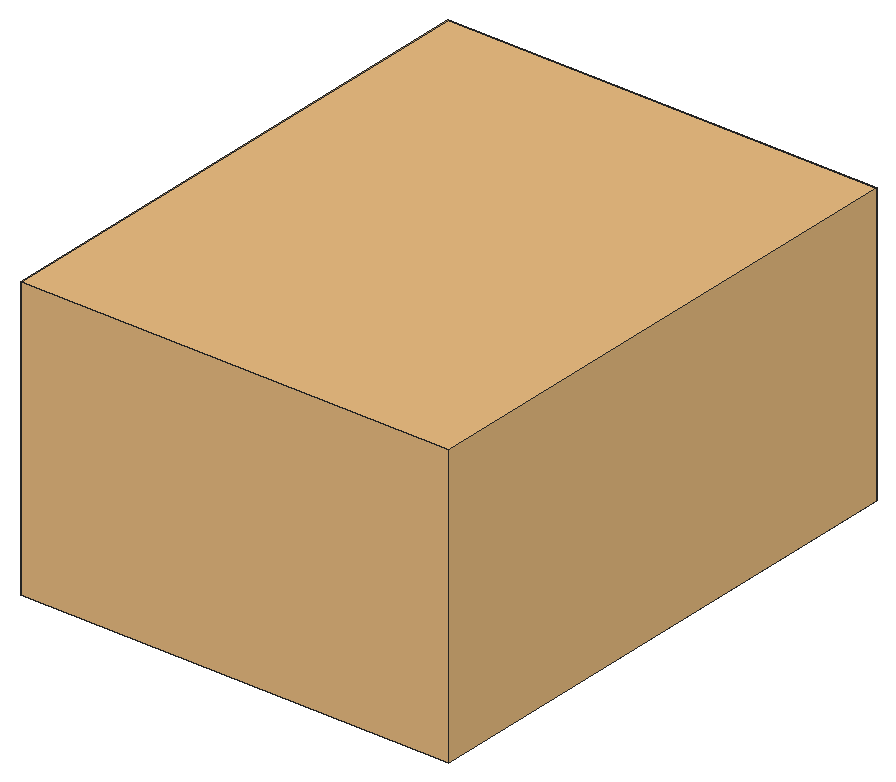
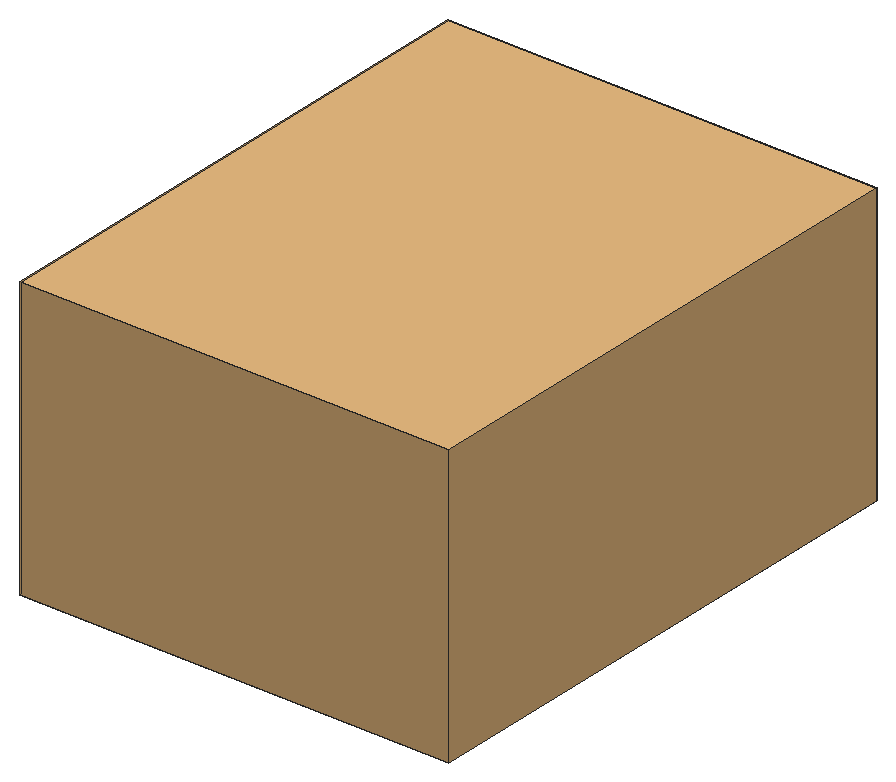
# SketchUp Ruby script. Lengths in inches.
U = 1.inch
M = Sketchup.active_model
def pt(a) = Geom::Point3d.new(a.map { |v| v * U })
def face(e, loops, mat)
  f = e.add_face(loops[0].map { |a| pt(a) })
  loops[1..].each { |l| e.add_face(l.map { |a| pt(a) }).erase! }
  f.material = f.back_material = mat if mat
  f
end
# faces: each face lists its corners as indices into pts; further lists are holes
def faces(e, pts, list, mat = nil) = list.each { |f| face(e, (f[0].is_a?(Array) ? f : [f]).map { |l| l.map { |i| pts[i] } }, mat) }
# xy, xz, yz: faces in a plane at the given z, y or x. An outline is a flat list of corners, or four numbers for a rectangle; further outlines are holes
def ring(l) = l.size == 4 ? [[l[0], l[1]], [l[2], l[1]], [l[2], l[3]], [l[0], l[3]]] : l.each_slice(2).to_a
def flat(e, list, mat, &to3) = list.each { |f| face(e, (f[0].is_a?(Array) ? f : [f]).map { |l| ring(l).map { |u, v| to3.(u, v) } }, mat) }
def xy(e, z, list, mat = nil) = flat(e, list, mat) { |x, y| [x, y, z] }
def xz(e, y, list, mat = nil) = flat(e, list, mat) { |x, z| [x, y, z] }
def yz(e, x, list, mat = nil) = flat(e, list, mat) { |y, z| [x, y, z] }
def lines(e, pts, list) = list.each { |a, b| e.add_line(pt(pts[a]), pt(pts[b])) }
# prism: a flat outline (further loops are holes) pulled along v
def prism(e, loops, v, mat = nil)
  f = face(e, loops, mat); d = Geom::Vector3d.new(v.map { |x| x * U })
  f.pushpull(f.normal.samedirection?(d) ? d.length : -d.length)
end
def box(e, o, s, mat = nil) = prism(e, [[o, [o[0] + s[0], o[1], o[2]], [o[0] + s[0], o[1] + s[1], o[2]], [o[0], o[1] + s[1], o[2]]]], [0, 0, s[2]], mat)
def at(x, y, z, deg = 0) = Geom::Transformation.translation(pt([x, y, z])) * Geom::Transformation.rotation(ORIGIN, Z_AXIS, deg.degrees)
def axes(o, x, y, z) = Geom::Transformation.new([*x, 0, *y, 0, *z, 0, *pt(o).to_a, 1])
def part(name) = M.definitions.add(name)
# library, detail: a bought-in or finely detailed component or shape, given as its bounding box
def library(name, o, s) = part(name).tap { |d| box(d.entities, o, s) }
def detail(e, o, s) = box(e.add_group.entities, o, s)
def put(e, d, t, mat = nil) = e.add_instance(d, t).tap { |i| i.material = mat if mat }
def group(e, t, mat = nil) = e.add_group.tap { |g| g.transformation = t; g.material = mat if mat }.entities
root = M.entities
M.materials.add("D02_Buttercup_Glow").color = [255, 229, 155]
M.materials.add("LightPink_Translucent").color = [144, 107, 117]
c1 = part("blade")
p = [[2.15,0.21,22],[0,0.17,0],[0.09,0.45,0],[2.18,0.31,22],[2.29,0.31,22],[0.38,0.45,0],
  [2.48,0.24,33],[2.49,0.24,33],[2.48,0.22,33]]
faces(c1.entities,p,[[0,1,2,3],[4,5,2,3],[6,3,4,7],[8,0,3,6]])
c2 = part("seeds")
p = [[0.3,-0.1,1.38],[-0.01,-0.03,1.59],[-0.01,-0.03,0.03],[0.14,-0.07,-0.07],[0.29,-0.03,3],[0.15,0.01,3.11]]
faces(c2.entities,p,[[0,1,2,3],[1,0,4,5]],"LightPink_Translucent")
c3 = part("blade with seeds")
put(c3.entities,c1,at(0,0,0))
put(c3.entities,c2,axes([2.4,0.25,30.99],[1.5799,-0.05474,1.17369],[-0.12525,1.92788,0.29478],[-0.07173,-0.02425,1.56792]))
c4 = library("Group\#1",[297.81,-2,0],[578,722,378])
put(root,c3,axes([77.12,76.59,44.18],[1.2866,-0.3514,-0.19198],[0.45209,1.01223,0.00008],[0.14202,-0.03884,1.73897]))
put(root,c3,axes([65.8,73.25,44.06],[1.27479,0.1698,-0.62353],[-0.26901,1.04736,-0.16365],[0.38043,0.12691,1.37633]))
put(root,c3,axes([77.8,73.25,44.06],[1.27479,0.1698,-0.62353],[-0.26901,1.04736,-0.16365],[0.38043,0.12691,1.37633]))
put(root,c3,axes([64.37,75.88,44.46],[-1.19666,-0.83357,-0.25192],[1.00694,-0.93603,0.5513],[-0.32224,0.09751,1.68216]))
put(root,c3,axes([76.37,75.88,44.46],[-1.19666,-0.83357,-0.25192],[1.00694,-0.93603,0.5513],[-0.32224,0.09751,1.68216]))
put(root,c3,axes([65.14,73.58,44.21],[0.73619,0.86927,-0.44739],[-1.11511,0.61213,0.21531],[0.23824,0.10756,1.43643]))
put(root,c3,axes([77.14,73.58,44.21],[0.73619,0.86927,-0.44739],[-1.11511,0.61213,0.21531],[0.23824,0.10756,1.43643]))
put(root,c3,axes([63.76,75.7,44.21],[-1.33077,0.06393,-0.44739],[-0.12035,-1.06125,0.21531],[-0.23824,0.10756,1.43643]))
put(root,c3,axes([75.76,75.7,44.21],[-1.33077,0.06393,-0.44739],[-0.12035,-1.06125,0.21531],[-0.23824,0.10756,1.43643]))
put(root,c3,axes([64.89,78.03,44.03],[-1.14332,-0.25625,-0.30978],[0.28787,-0.90242,0.30978],[-0.23049,0.10406,1.38974]))
put(root,c3,axes([76.89,78.03,44.03],[-1.14332,-0.25625,-0.30978],[0.28787,-0.90242,0.30978],[-0.23049,0.10406,1.38974]))
put(root,c3,axes([65.38,74.18,44.67],[1.38012,0.49416,-0.29095],[-0.66454,1.04299,-0.50002],[0.04337,0.25608,1.59708]))
put(root,c3,axes([77.38,74.18,44.67],[1.38012,0.49416,-0.29095],[-0.66454,1.04299,-0.50002],[0.04337,0.25608,1.59708]))
put(root,c3,axes([68.38,75.35,44.03],[-0.85545,0.64616,-0.30978],[-0.85545,-0.64616,0.30978],[0,0.20813,1.38974]))
put(root,c3,axes([80.38,75.35,44.03],[-0.85545,0.64616,-0.30978],[-0.85545,-0.64616,0.30978],[0,0.20813,1.38974]))
put(root,c3,axes([64.69,75.42,44.67],[0.1428,1.18174,-0.29095],[-1.48733,0.07145,-0.50002],[-0.26191,0.15741,1.59708]))
put(root,c3,axes([76.69,75.42,44.67],[0.1428,1.18174,-0.29095],[-1.48733,0.07145,-0.50002],[-0.26191,0.15741,1.59708]))
put(root,c3,axes([65.24,74.95,44.21],[-0.59459,0.93321,-0.44739],[-1.23546,-0.44912,0.21531],[0,0.21512,1.43643]))
put(root,c3,axes([77.24,74.95,44.21],[-0.59459,0.93321,-0.44739],[-1.23546,-0.44912,0.21531],[0,0.21512,1.43643]))
put(root,c3,axes([63.8,76.32,44.06],[-0.82544,0.77843,-0.62353],[-1.0254,-0.70586,-0.16365],[-0.33076,0.19418,1.37633]))
put(root,c3,axes([75.8,76.32,44.06],[-0.82544,0.77843,-0.62353],[-1.0254,-0.70586,-0.16365],[-0.33076,0.19418,1.37633]))
put(root,c3,axes([65.16,78.44,44.02],[-1.14694,0.51783,-0.49651],[-0.68554,-0.92854,0],[-0.26122,0.11794,1.57504]))
put(root,c3,axes([77.16,78.44,44.02],[-1.14694,0.51783,-0.49651],[-0.68554,-0.92854,0],[-0.26122,0.11794,1.57504]))
put(root,c3,axes([68.97,75.38,44.02],[0,1.03566,-0.49651],[-1.37109,0,0],[0,0.23588,1.57504]))
put(root,c3,axes([80.97,75.38,44.02],[0,1.03566,-0.49651],[-1.37109,0,0],[0,0.23588,1.57504]))
put(root,c3,axes([67.42,78.63,43.49],[0.08928,-0.14952,1.76342],[1.12407,-0.44035,-0.26939],[0.34078,0.22791,0.30037]))
put(root,c3,axes([79.42,78.63,43.49],[0.08928,-0.14952,1.76342],[1.12407,-0.44035,-0.26939],[0.34078,0.22791,0.30037]))
put(root,c3,axes([65.94,75.24,44.09],[0.44936,0.94823,-0.69212],[-1.29441,0.3415,-0.18165],[0.04967,0.32109,1.52773]))
put(root,c3,axes([77.94,75.24,44.09],[0.44936,0.94823,-0.69212],[-1.29441,0.3415,-0.18165],[0.04967,0.32109,1.52773]))
put(root,c3,axes([57.1,78.51,43.49],[0.16438,0.10347,1.76342],[0.27873,0.95868,-0.26939],[-0.36432,0.20444,0.30037]))
put(root,c3,axes([69.1,78.51,43.49],[0.16438,0.10347,1.76342],[0.27873,0.95868,-0.26939],[-0.36432,0.20444,0.30037]))
put(root,c3,axes([62.17,78.6,43.49],[0.19833,-0.05635,1.76342],[1.19302,0.31018,-0.26939],[0.03489,0.3496,0.30037]))
put(root,c3,axes([74.17,78.6,43.49],[0.19833,-0.05635,1.76342],[1.19302,0.31018,-0.26939],[0.03489,0.3496,0.30037]))
put(root,c4,at(-770.92,3.11,-6),"D02_Buttercup_Glow")
put(root,c3,axes([72.59,385.52,32.11],[0.28013,0.33252,1.71376],[-1.29445,0.27994,0.13857],[-0.29256,-0.52202,0.73262]))
put(root,c3,axes([74.73,383.31,32.95],[-0.18744,-0.14521,1.74944],[-1.25089,0.09206,-0.27667],[-0.19964,-0.34731,0.14031]))
put(root,c3,axes([77.625,385.04,30.83],[-0.34835,0.20963,1.43002],[-1.04325,-0.36691,-0.30754],[0.19338,-0.4563,0.61141]))
put(root,c3,axes([76.04,385.77,33.22],[-0.5849,-0.8421,-0.71045],[1.20401,-0.4693,0.08574],[-0.13677,-0.40688,1.00501]))
put(root,c3,axes([72.23,384.64,30.83],[-0.07421,0.33879,1.43002],[-1.08488,0.28361,-0.30754],[-0.25359,-0.4379,0.61141]))
put(root,c3,axes([75.03,383.9,29.73],[-0.20555,0.03731,1.76342],[-1.13672,-0.42002,-0.26939],[0.01907,-0.35034,0.30037]))
put(root,c3,axes([78.47,386.59,33.22],[0.03189,-0.95798,-0.71045],[1.34277,0.06434,0.08574],[0.14171,-0.40585,1.00501]))
put(root,c3,axes([80.35,385.09,32.95],[-0.01183,-0.20612,1.74944],[-0.99913,-0.59572,-0.27667],[0.15447,-0.36112,0.14031]))
put(root,c3,axes([76.15,385.05,32.76],[0.36946,-0.79643,-0.35414],[1.07787,0.23229,0.4572],[-0.09883,-0.32066,0.87481]))
put(root,c3,axes([76.96,386.11,32.11],[-0.22818,0.35597,1.71376],[-0.95725,-0.73667,0.13857],[0.43183,-0.45914,0.73262]))
put(root,c3,axes([80.08,384.35,32.95],[-0.12446,0.07911,1.77383],[-1.21937,-0.26689,-0.16761],[-0.04414,-0.34521,0.31391]))
put(root,c3,axes([75.6,385.6,32.92],[-1.20468,-0.25962,-0.51099],[0.41292,-0.89013,-0.3958],[-0.11046,-0.35838,0.97773]))
put(root,c3,axes([76.34,383.37,31],[0.15721,0.60392,1.1486],[-0.87211,-0.33448,0.84392],[0.09385,-0.30923,0.25299]))
put(root,c3,axes([78.2,386.27,32.92],[-0.87728,-0.69587,-0.51099],[0.92674,-0.60943,-0.3958],[0.13348,-0.35356,0.97773]))
put(root,c3,axes([73.44,382.84,32.95],[-0.02286,0.12414,1.77383],[-1.12758,0.45052,-0.16761],[-0.33182,-0.23029,0.31391]))
put(root,c3,axes([73.2,385.04,33.33],[1.36515,-0.26619,0.53763],[0.23692,1.04421,0.4433],[-0.32106,-0.30775,1.11249]))
put(root,c3,axes([76.28,385.24,32.97],[1.20755,0.27075,0.48003],[-0.41292,0.89013,0.3958],[-0.07257,-0.35005,0.9933]))
put(root,c3,axes([76.63,385.56,33.27],[-1.19922,0.48218,-0.1216],[-0.58932,-0.85579,-0.67495],[-0.15822,-0.36063,1.02557]))
put(root,c3,axes([79.12,386.64,33.27],[-1.34686,-0.05131,-0.1216],[0.03681,-0.97156,-0.67495],[0.09356,-0.37418,1.02557]))
put(root,c3,axes([79.03,386.01,32.76],[0.82919,-0.54528,-0.35414],[0.78493,0.62262,0.4572],[0.11943,-0.31634,0.87481]))
put(root,c3,axes([71.86,384.09,31],[0.63926,0.36046,1.1486],[-0.93099,0.21668,0.84392],[-0.1992,-0.27702,0.25299]))
put(root,c3,axes([76.6,385.17,32.97],[0.90301,-0.35198,0.0643],[0.44199,0.64184,0.50621],[-0.08721,-0.28293,0.77189]))
put(root,c3,axes([73.4,386.01,33.22],[-1.04497,-0.50058,-0.71045],[0.74264,-0.8772,0.08574],[-0.3786,-0.29889,1.00501]))
put(root,c3,axes([73.04,385.34,32.76],[-0.18927,-0.83419,-0.35414],[1.08199,-0.22027,0.4572],[-0.29062,-0.23905,0.87481]))
put(root,c3,axes([73.51,385.27,32.97],[0.55698,-0.6579,0.0643],[0.79316,0.38303,0.50621],[-0.25643,-0.21093,0.77189]))
put(root,c3,axes([71.35,385.18,29.73],[-0.11871,0.13643,1.76342],[-1.19964,0.29415,-0.26939],[-0.2898,-0.26759,0.30037]))
put(root,c3,axes([34.1875,387.14,43.49],[-0.20555,0.03731,1.76342],[-1.13672,-0.42002,-0.26939],[0.01907,-0.35034,0.30037]))
put(root,c3,axes([73.33,388.93,30.33],[-0.50328,-1.06202,-0.69835],[1.44974,-0.38248,-0.18329],[-0.05563,-0.35963,1.54149]))
put(root,c3,axes([70.71,386.56,32.11],[0.45521,0.17844,1.71376],[-0.94204,0.74856,0.13857],[-0.58713,-0.33769,0.73262]))
put(root,c3,axes([80.0625,385.69,29.73],[-0.18342,-0.08159,1.76342],[-0.47115,-0.9115,-0.26939],[0.31784,-0.24736,0.30037]))
put(root,c3,axes([76.27,385.89,33.29],[-0.36946,0.79643,0.35414],[-1.07787,-0.23229,-0.4572],[-0.09883,-0.32066,0.87481]))
put(root,c3,axes([72.91,386.03,32.92],[-1.20928,0.24619,-0.51099],[-0.21154,-0.93233,-0.3958],[-0.32481,-0.26718,0.97773]))
put(root,c3,axes([79.02,386.23,32.97],[0.87265,0.70663,0.48003],[-0.92674,0.60943,0.3958],[0.16097,-0.33153,0.9933]))
put(root,c3,axes([73.76,385.2,33.67],[-0.81789,0.99285,-0.13619],[-1.18445,-0.572,-0.75594],[-0.41173,-0.28051,1.14864]))
put(root,c3,axes([79.35,386.29,32.97],[1.00708,0.04826,0.0643],[-0.02761,0.72867,0.50621],[0.10538,-0.27912,0.77189]))
put(root,c3,axes([78.59,386.79,33.29],[-0.82919,0.54528,0.35414],[-0.78493,-0.62262,-0.4572],[0.11943,-0.31634,0.87481]))
put(root,c3,axes([80.06,388.26,33.22],[0.64013,-0.81717,-0.71045],[1.12174,0.58074,0.08574],[0.38221,-0.29607,1.00501]))
put(root,c3,axes([73.14,385.875,30.61],[-0.7662,-1.03778,0],[1.28187,-0.57875,-0.51607],[0.29196,-0.13181,1.63711]))
put(root,c3,axes([80.02,387.875,32.92],[-0.31482,-0.94565,-0.51099],[1.19224,-0.16542,-0.3958],[0.34166,-0.254,0.97773]))
put(root,c3,axes([74.82,384.625,30.36],[-0.84686,0.59414,-0.03893],[-0.77596,-0.65071,-0.17649],[-0.05463,-0.18438,0.58215]))
put(root,c3,axes([70.625,384.91,32.95],[-0.26368,-0.00731,1.74944],[-0.83946,0.73103,-0.27667],[-0.44791,-0.14937,0.14031]))
put(root,c3,axes([80.59,388.55,33.27],[-1.1336,-0.57106,-0.1216],[0.65308,-0.827,-0.67495],[0.32027,-0.28747,1.02557]))
put(root,c3,axes([75.9,391.67,31.5625],[1.05902,0.41762,1.51261],[-1.03748,0.89969,0.59816],[-0.46471,-0.53324,1.26806]))
put(root,c3,axes([73.68,386.02,33.29],[0.18927,0.83419,0.35414],[-1.08199,0.22027,-0.4572],[-0.29062,-0.23905,0.87481]))
put(root,c3,axes([70.37,388.78,30.25],[0,-1.03566,-0.49651],[1.37109,0,0],[0,-0.23588,1.57504]))
put(root,c3,axes([74.18,385.72,30.25],[1.14694,-0.51783,-0.49651],[0.68554,0.92854,0],[0.26122,-0.11794,1.57504]))
put(root,c3,axes([80.98,387.51,30.83],[-0.4378,-0.03068,1.43002],[-0.44851,-0.8229,-0.30754],[0.53783,-0.23279,0.61141]))
put(root,c3,axes([70.43,386.57,33.33],[1.01205,-0.7643,0.53763],[0.87284,0.81167,0.4433],[-0.47482,-0.14098,1.11249]))
put(root,c3,axes([83.38,388.3,32.95],[-0.16006,-0.00787,1.77383],[-0.66468,-0.8428,-0.16761],[0.26693,-0.27711,0.31391]))
put(root,c3,axes([75.54,387.84,30.3],[0.82544,-0.77843,-0.62353],[1.0254,0.70586,-0.16365],[0.33076,-0.19418,1.37633]))
put(root,c3,axes([81.49,385.99,31],[-0.40819,0.5272,1.1486],[-0.35086,-0.70831,0.84392],[0.33713,-0.17749,0.25299]))
put(root,c3,axes([80.9,387.97,32.76],[1.06674,-0.14801,-0.35414],[0.28168,0.84611,0.4572],[0.30569,-0.22726,0.87481]))
put(root,c3,axes([30.51,388.42,43.49],[-0.11871,0.13643,1.76342],[-1.19964,0.29415,-0.26939],[-0.2898,-0.26759,0.30037]))
put(root,c3,axes([70.89,386.5625,32.97],[0.06171,-0.78753,0.0643],[0.9318,0.02159,0.50621],[-0.35694,-0.08241,0.77189]))
put(root,c3,axes([32.49,392.17,44.1],[-0.50328,-1.06202,-0.69835],[1.44974,-0.38248,-0.18329],[-0.05563,-0.35963,1.54149]))
put(root,c3,axes([74.1,389.2,30.45],[0.59459,-0.93321,-0.44739],[1.23546,0.44912,0.21531],[0,-0.21512,1.43643]))
put(root,c3,axes([70.54,386.8125,32.76],[-0.69728,-0.64842,-0.35414],[0.79619,-0.61382,0.4572],[-0.40453,-0.09339,0.87481]))
put(root,c3,axes([39.22,388.93,43.49],[-0.18342,-0.08159,1.76342],[-0.47115,-0.9115,-0.26939],[0.31784,-0.24736,0.30037]))
put(root,c3,axes([74.64,388.74,30.9],[-0.1428,-1.18174,-0.29095],[1.48733,-0.07145,-0.50002],[0.26191,-0.15741,1.59708]))
put(root,c3,axes([70.95,388.8,30.26],[0.85545,-0.64616,-0.30978],[0.85545,0.64616,0.30978],[0,-0.20813,1.38974]))
put(root,c3,axes([70.61,385.71,30.36],[-0.35352,0.84566,-0.03893],[-1.08806,-0.26014,-0.17649],[-0.1652,-0.13832,0.58215]))
put(root,c3,axes([80.03,388.47,33.29],[-1.06674,0.14801,0.35414],[-0.28168,-0.84611,-0.4572],[0.30569,-0.22726,0.87481]))
put(root,c3,axes([73.95,389.98,30.9],[-1.38012,-0.49416,-0.29095],[0.66454,-1.04299,-0.50002],[-0.04337,-0.25608,1.59708]))
put(root,c3,axes([70.02,389.57,30.61],[-1.53239,0,0],[0,-1.1575,-0.51607],[0,-0.26363,1.63711]))
put(root,c3,axes([70.29,387.5,30.83],[0.23927,0.28834,1.43002],[-0.55135,0.78376,-0.30754],[-0.56612,-0.18733,0.61141]))
put(root,c3,axes([74.45,386.125,30.26],[1.14332,0.25625,-0.30978],[-0.28787,0.90242,0.30978],[0.23049,-0.10406,1.38974]))
put(root,c3,axes([71.27,387.24,33.22],[-1.22504,-0.02494,-0.71045],[0.08228,-1.05005,0.08574],[-0.51899,-0.11081,1.00501]))
put(root,c3,axes([33.98,387.87,44.13],[-0.84686,0.59414,-0.03893],[-0.77596,-0.65071,-0.17649],[-0.05463,-0.18438,0.58215]))
put(root,c3,axes([81,388.34,32.97],[0.8413,0.43556,0.0643],[-0.48981,0.62025,0.50621],[0.26973,-0.20053,0.77189]))
put(root,c3,axes([80.77,388.16,32.97],[0.30393,0.95317,0.48003],[-1.19224,0.16542,0.3958],[0.35138,-0.22417,0.9933]))
put(root,c3,axes([83.98,389.31,32.95],[0.17006,-0.15775,1.74944],[-0.21766,-0.96766,-0.27667],[0.42669,-0.18347,0.14031]))
put(root,c3,axes([71.21,389.26,30.57],[-1.1399,0.87071,0.30756],[-1.1406,-0.86155,-0.36492],[-0.03981,-0.24727,1.64885]))
put(root,c3,axes([69.61,385.53,32.95],[0.09085,0.10335,1.77383],[-0.43798,0.92907,-0.16761],[-0.44357,0.00672,0.31391]))
put(root,c3,axes([74.84,389.67,30.67],[1.3808,0.50196,0.24065],[-0.66454,1.04299,0.50002],[0,-0.24043,1.60543]))
put(root,c3,axes([29.53,392.02,44.02],[0,-1.03566,-0.49651],[1.37109,0,0],[0,-0.23588,1.57504]))
put(root,c3,axes([33.34,388.96,44.02],[1.14694,-0.51783,-0.49651],[0.68554,0.92854,0],[0.26122,-0.11794,1.57504]))
put(root,c3,axes([74.3,391.08,30.68],[0.32481,-1.2272,-0.23429],[1.54007,0.21392,0.51271],[-0.26911,-0.16947,1.5644]))
put(root,c3,axes([70.87,387.46,32.92],[-0.88986,0.68603,-0.51099],[-0.77932,-0.72471,-0.3958],[-0.45212,-0.10438,0.97773]))
put(root,c3,axes([71.53,387.15,33.29],[0.69728,0.64842,0.35414],[-0.79619,0.61382,-0.4572],[-0.40453,-0.09339,0.87481]))
put(root,c3,axes([34.7,391.08,44.06],[0.82544,-0.77843,-0.62353],[1.0254,0.70586,-0.16365],[0.33076,-0.19418,1.37633]))
put(root,c3,axes([68.86,388.37,31],[0.78239,-0.07411,1.1486],[-0.49629,0.65296,0.84392],[-0.38663,-0.09795,0.25299]))
put(root,c3,axes([74.39,388.97,30.95],[-1.33077,0.06393,0.44739],[-0.12035,-1.06125,-0.21531],[0.23824,-0.10756,1.43643]))
put(root,c3,axes([71.33,386.74,33.27],[-0.06562,1.05324,-0.1216],[-1.2424,-0.02879,-0.67495],[-0.4785,-0.07316,1.02557]))
put(root,c3,axes([70.95,389.74,30.71],[0,1.03566,0.49651],[-1.37109,0,0],[0,-0.23588,1.57504]))
put(root,c3,axes([80.63,390.78,33.27],[-0.6166,-0.93779,-0.1216],[1.09436,-0.46085,-0.67495],[0.46117,-0.12373,1.02557]))
put(root,c3,axes([80.58,389.97,32.92],[0.332,-0.94205,-0.51099],[1.13828,0.3229,-0.3958],[0.45829,-0.08638,0.97773]))
put(root,c3,axes([78.78,386.14,30.61],[0.7662,-1.03778,0],[1.28187,0.57875,-0.51607],[0.29196,0.13181,1.63711]))
put(root,c3,axes([69.75,388.1875,32.11],[0.50831,-0.02346,1.71376],[-0.33721,1.01661,0.13857],[-0.72439,-0.06288,0.73262]))
put(root,c3,axes([74.19,390.58,30.45],[-0.73619,-0.86927,-0.44739],[1.11511,-0.61213,0.21531],[-0.23824,-0.10756,1.43643]))
put(root,c3,axes([74.34,389.35,30.6],[0.53281,1.15808,0.45755],[-1.52239,0.4027,0.17955],[0.01861,-0.2128,1.58856]))
put(root,c3,axes([33.26,392.44,44.21],[0.59459,-0.93321,-0.44739],[1.23546,0.44912,0.21531],[0,-0.21512,1.43643]))
put(root,c3,axes([33.8,391.98,44.67],[-0.1428,-1.18174,-0.29095],[1.48733,-0.07145,-0.50002],[0.26191,-0.15741,1.59708]))
put(root,c3,axes([30.11,392.05,44.03],[0.85545,-0.64616,-0.30978],[0.85545,0.64616,0.30978],[0,-0.20813,1.38974]))
put(root,c3,axes([81.79,390.24,30.22],[-0.7893,0.12429,1.41583],[-0.12563,-0.9893,0.08104],[0.55282,-0.14974,0.80566]))
put(root,c3,axes([83.23,389.36,30.5],[-0.75977,-0.66224,-0.06488],[0.83212,-0.6068,-0.29416],[0.23578,-0.04272,0.97024]))
put(root,c3,axes([29.77,388.95,44.13],[-0.35352,0.84566,-0.03893],[-1.08806,-0.26014,-0.17649],[-0.1652,-0.13832,0.58215]))
put(root,c3,axes([74.08,390.26,30.95],[-0.59459,0.93321,0.44739],[-1.23546,-0.44912,-0.21531],[0,-0.21512,1.43643]))
put(root,c3,axes([33.11,393.22,44.67],[-1.38012,-0.49416,-0.29095],[0.66454,-1.04299,-0.50002],[-0.04337,-0.25608,1.59708]))
put(root,c3,axes([76.26,389.45,30.44],[0,-1.19833,0],[1.53239,0,0],[0,0,1.79456]))
put(root,c3,axes([78.12,386.68,30.71],[-1.14694,-0.51783,0.49651],[0.68554,-0.92854,0],[0.26122,0.11794,1.57504]))
put(root,c3,axes([80.36,390.32,33.22],[1.07686,-0.45739,-0.71045],[0.60013,0.94154,0.08574],[0.52031,-0.10696,1.00501]))
put(root,c3,axes([33.6,389.37,44.03],[1.14332,0.25625,-0.30978],[-0.28787,0.90242,0.30978],[0.23049,-0.10406,1.38974]))
put(root,c3,axes([73.53,390.91,30.3],[-1.27479,-0.1698,-0.62353],[0.26901,-1.04736,-0.16365],[-0.38043,-0.12691,1.37633]))
put(root,c3,axes([75.53,388.69,30.6],[-1.01611,0.93987,0.45755],[-1.20717,-0.82966,0.17955],[0.24496,-0.0938,1.58856]))
put(root,c3,axes([76.64,390.38,30.53],[-1.1399,-0.8914,-0.06131],[1.1406,-0.89194,0],[-0.03981,-0.03113,1.75571]))
put(root,c3,axes([73.77,387.15,30.71],[-0.35402,1.02926,0.17642],[-1.29548,-0.29127,0.35086],[0.22379,-0.00501,1.60407]))
put(root,c3,axes([80.2,390.5,33.29],[-1.01846,-0.28891,0.35414],[0.29705,-0.84289,-0.4572],[0.41005,-0.07729,0.87481]))
put(root,c3,axes([69.54,388.96,32.97],[0.34623,-0.9443,0.48003],[1.13828,0.3229,0.3958],[-0.44763,0.05675,0.9933]))
put(root,c3,axes([73.23,387.98,29.83],[-1.20625,0.41464,1.28929],[-0.38394,-1.1897,0.50096],[0.74071,0.01979,1.46642]))
put(root,c3,axes([76.48,388.29,30.85],[0.23642,-0.92427,0.1448],[1.15506,0.16044,-0.41347],[0.21021,0.09491,1.26744]))
put(root,c3,axes([69.46,388.71,32.97],[-0.4501,-0.70615,0.0643],[0.82077,-0.34564,0.50621],[-0.36181,0.0682,0.77189]))
put(root,c3,axes([74.48,390.49,30.6],[1.54892,0.2182,0.45755],[-0.31522,1.23236,0.17955],[-0.22636,-0.119,1.58856]))
put(root,c3,axes([82.66,389.59,29.73],[-0.06405,-0.15723,1.76342],[0.44421,-0.91974,-0.26939],[0.4481,-0.01323,0.30037]))
put(root,c3,axes([69.43,389.43,29.73],[0.03108,0.16322,1.76342],[-0.62654,0.85237,-0.26939],[-0.44504,-0.04296,0.30037]))
put(root,c3,axes([75.98,388.53,30.95],[-0.73619,-0.86927,0.44739],[1.11511,-0.61213,-0.21531],[0.23824,0.10756,1.43643]))
put(root,c3,axes([72.18,392.51,30.26],[-0.28787,-0.90242,-0.30978],[1.14332,-0.25625,0.30978],[-0.23049,-0.10406,1.38974]))
put(root,c3,axes([33.46,394.32,44.4375],[0.32481,-1.2272,-0.23429],[1.54007,0.21392,0.51271],[-0.26911,-0.16947,1.5644]))
put(root,c3,axes([73.65,392.46,30.71],[1.31687,-0.27488,0.17642],[0.32517,1.02297,0.35086],[-0.11745,-0.14905,1.60407]))
put(root,c3,axes([76.36,388.59,30.9],[1.23732,-0.68758,-0.29095],[0.8228,0.97154,-0.50002],[0.30528,0.09867,1.59708]))
put(root,c3,axes([81.28,390.4,32.76],[1.01846,0.28891,-0.35414],[-0.29705,0.84289,0.4572],[0.41005,-0.07729,0.87481]))
put(root,c3,axes([71.86,392.89,30.25],[-1.14694,-0.51783,-0.49651],[0.68554,-0.92854,0],[-0.26122,-0.11794,1.57504]))
put(root,c3,axes([79.48,386.76,30.25],[1.14694,0.51783,-0.49651],[-0.68554,0.92854,0],[0.26122,0.11794,1.57504]))
put(root,c3,axes([69.31,389.0625,32.76],[-1.01846,-0.28891,-0.35414],[0.29705,-0.84289,0.4572],[-0.41005,0.07729,0.87481]))
put(root,c3,axes([77.3,389.72,30.44],[1.37109,0,0],[0,1.07219,0],[0,0,1.78407]))
put(root,c3,axes([74.98,391.07,30.9],[-1.23732,0.68758,-0.29095],[-0.8228,-0.97154,-0.50002],[-0.30528,-0.09867,1.59708]))
put(root,c3,axes([77.6875,387.2,30.71],[-1.31687,0.27488,0.17642],[-0.32517,-1.02297,0.35086],[0.11745,0.14905,1.60407]))
put(root,c3,axes([78.5,389.36,32.11],[-0.50831,0.02346,1.71376],[0.33721,-1.01661,0.13857],[0.72439,0.06288,0.73262]))
put(root,c3,axes([79.16,387.15,30.26],[0.28787,0.90242,-0.30978],[-1.14332,0.25625,0.30978],[0.23049,0.10406,1.38974]))
put(root,c3,axes([33.35,393.82,44.21],[-0.73619,-0.86927,-0.44739],[1.11511,-0.61213,0.21531],[-0.23824,-0.10756,1.43643]))
put(root,c3,axes([81.125,390.76,32.97],[0.4501,0.70615,0.0643],[-0.82077,0.34564,0.50621],[0.36181,-0.0682,0.77189]))
put(root,c3,axes([42.39,392.6,44.26],[-0.75977,-0.66224,-0.06488],[0.83212,-0.6068,-0.29416],[0.23578,-0.04272,0.97024]))
